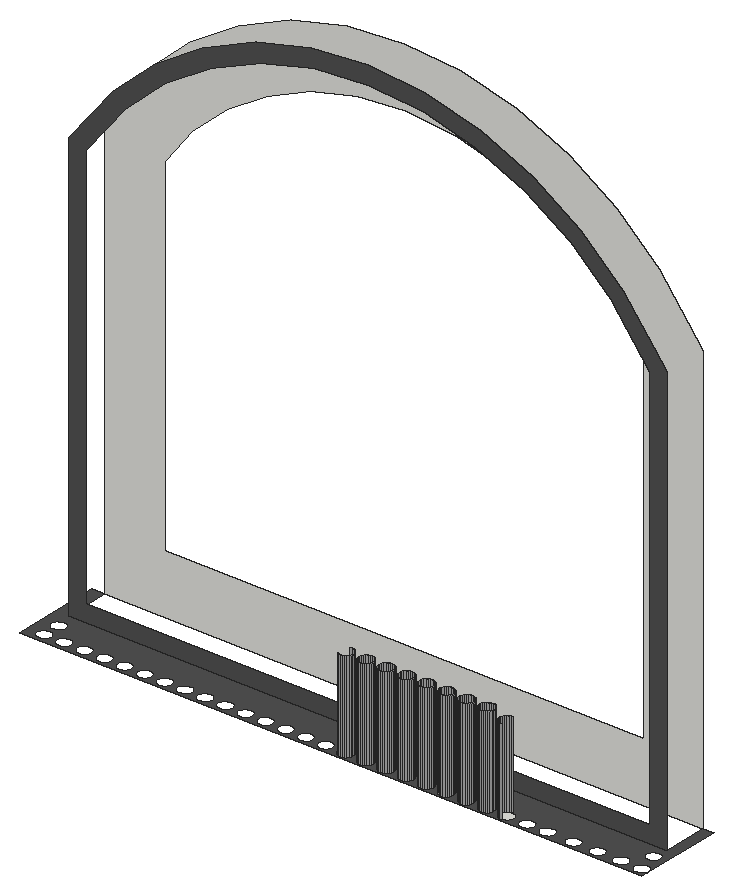
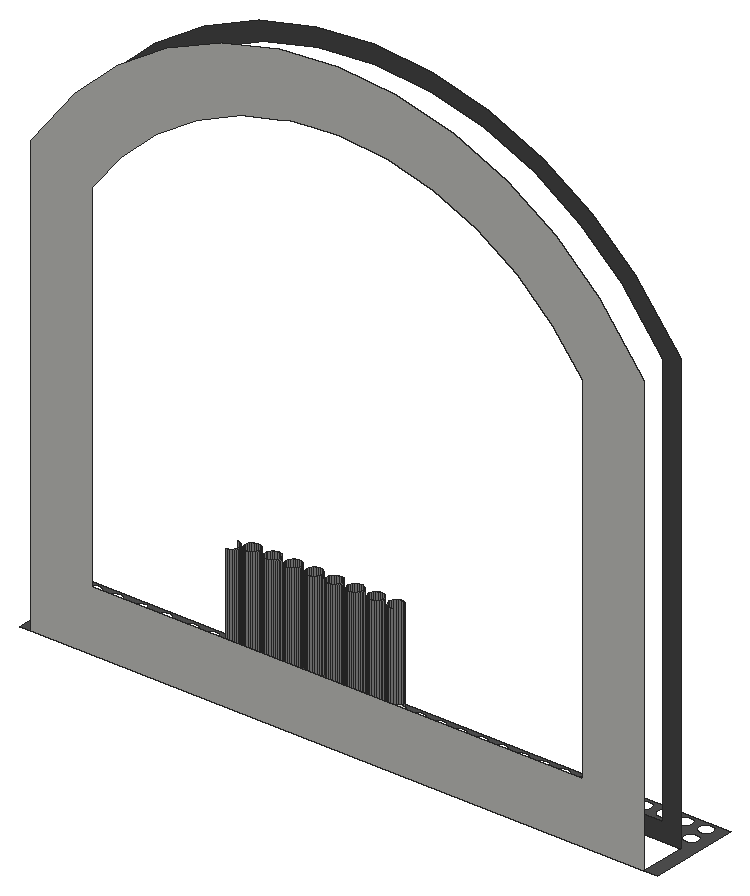
# SketchUp Ruby script. Lengths in inches.
U = 1.inch
M = Sketchup.active_model
def pt(a) = Geom::Point3d.new(a.map { |v| v * U })
def face(e, loops, mat)
  f = e.add_face(loops[0].map { |a| pt(a) })
  loops[1..].each { |l| e.add_face(l.map { |a| pt(a) }).erase! }
  f.material = f.back_material = mat if mat
  f
end
# faces: each face lists its corners as indices into pts; further lists are holes
def faces(e, pts, list, mat = nil) = list.each { |f| face(e, (f[0].is_a?(Array) ? f : [f]).map { |l| l.map { |i| pts[i] } }, mat) }
# xy, xz, yz: faces in a plane at the given z, y or x. An outline is a flat list of corners, or four numbers for a rectangle; further outlines are holes
def ring(l) = l.size == 4 ? [[l[0], l[1]], [l[2], l[1]], [l[2], l[3]], [l[0], l[3]]] : l.each_slice(2).to_a
def flat(e, list, mat, &to3) = list.each { |f| face(e, (f[0].is_a?(Array) ? f : [f]).map { |l| ring(l).map { |u, v| to3.(u, v) } }, mat) }
def xy(e, z, list, mat = nil) = flat(e, list, mat) { |x, y| [x, y, z] }
def xz(e, y, list, mat = nil) = flat(e, list, mat) { |x, z| [x, y, z] }
def yz(e, x, list, mat = nil) = flat(e, list, mat) { |y, z| [x, y, z] }
def lines(e, pts, list) = list.each { |a, b| e.add_line(pt(pts[a]), pt(pts[b])) }
# prism: a flat outline (further loops are holes) pulled along v
def prism(e, loops, v, mat = nil)
  f = face(e, loops, mat); d = Geom::Vector3d.new(v.map { |x| x * U })
  f.pushpull(f.normal.samedirection?(d) ? d.length : -d.length)
end
def box(e, o, s, mat = nil) = prism(e, [[o, [o[0] + s[0], o[1], o[2]], [o[0] + s[0], o[1] + s[1], o[2]], [o[0], o[1] + s[1], o[2]]]], [0, 0, s[2]], mat)
def at(x, y, z, deg = 0) = Geom::Transformation.translation(pt([x, y, z])) * Geom::Transformation.rotation(ORIGIN, Z_AXIS, deg.degrees)
def axes(o, x, y, z) = Geom::Transformation.new([*x, 0, *y, 0, *z, 0, *pt(o).to_a, 1])
def part(name) = M.definitions.add(name)
# library, detail: a bought-in or finely detailed component or shape, given as its bounding box
def library(name, o, s) = part(name).tap { |d| box(d.entities, o, s) }
def detail(e, o, s) = box(e.add_group.entities, o, s)
def put(e, d, t, mat = nil) = e.add_instance(d, t).tap { |i| i.material = mat if mat }
def group(e, t, mat = nil) = e.add_group.tap { |g| g.transformation = t; g.material = mat if mat }.entities
root = M.entities
M.materials.add("[0132_LightGray]").color = [169, 169, 169]
M.materials.add("[0135_DarkGray]").color = [81, 81, 81]
xy(root,180.28,[[302.06,32.09,301.6875,32.13,301.34,32.28,301.04,32.51,300.8125,32.8,300.67,33.15,300.62,33.52,300.67,33.89,300.8125,34.24,301.04,34.54,301.34,34.77,301.6875,34.91,302.06,34.96,302.43,34.91,302.78,34.77,303.08,34.54,303.3,34.24,303.45,33.89,303.5,33.52,303.45,33.15,303.3,32.8,303.08,32.51,302.78,32.28,302.43,32.13],[306.12,32.09,305.75,32.13,305.4,32.28,305.1,32.51,304.875,32.8,304.73,33.15,304.68,33.52,304.73,33.89,304.875,34.24,305.1,34.54,305.4,34.77,305.75,34.91,306.12,34.96,306.49,34.91,306.84,34.77,307.14,34.54,307.37,34.24,307.51,33.89,307.56,33.52,307.51,33.15,307.37,32.8,307.14,32.51,306.84,32.28,306.49,32.13],[310.18,32.09,309.8125,32.13,309.47,32.28,309.17,32.51,308.9375,32.8,308.8,33.15,308.75,33.52,308.8,33.89,308.9375,34.24,309.17,34.54,309.47,34.77,309.8125,34.91,310.18,34.96,310.56,34.91,310.9,34.77,311.2,34.54,311.43,34.24,311.57,33.89,311.62,33.52,311.57,33.15,311.43,32.8,311.2,32.51,310.9,32.28,310.56,32.13],[314.25,32.09,313.875,32.13,313.53,32.28,313.23,32.51,313,32.8,312.86,33.15,312.81,33.52,312.86,33.89,313,34.24,313.23,34.54,313.53,34.77,313.875,34.91,314.25,34.96,314.62,34.91,314.97,34.77,315.26,34.54,315.49,34.24,315.63,33.89,315.68,33.52,315.63,33.15,315.49,32.8,315.26,32.51,314.97,32.28,314.62,32.13],[318.31,32.09,317.9375,32.13,317.59,32.28,317.29,32.51,317.0625,32.8,316.92,33.15,316.87,33.52,316.92,33.89,317.0625,34.24,317.29,34.54,317.59,34.77,317.9375,34.91,318.31,34.96,318.68,34.91,319.03,34.77,319.33,34.54,319.55,34.24,319.7,33.89,319.75,33.52,319.7,33.15,319.55,32.8,319.33,32.51,319.03,32.28,318.68,32.13],
  [322.37,32.09,322,32.13,321.65,32.28,321.35,32.51,321.125,32.8,320.98,33.15,320.93,33.52,320.98,33.89,321.125,34.24,321.35,34.54,321.65,34.77,322,34.91,322.37,34.96,322.74,34.91,323.09,34.77,323.39,34.54,323.62,34.24,323.76,33.89,323.81,33.52,323.76,33.15,323.62,32.8,323.39,32.51,323.09,32.28,322.74,32.13],[326.43,32.09,326.0625,32.13,325.72,32.28,325.42,32.51,325.1875,32.8,325.05,33.15,325,33.52,325.05,33.89,325.1875,34.24,325.42,34.54,325.72,34.77,326.0625,34.91,326.43,34.96,326.81,34.91,327.15,34.77,327.45,34.54,327.68,34.24,327.82,33.89,327.87,33.52,327.82,33.15,327.68,32.8,327.45,32.51,327.15,32.28,326.81,32.13],[330.5,32.09,330.125,32.13,329.78,32.28,329.48,32.51,329.25,32.8,329.11,33.15,329.06,33.52,329.11,33.89,329.25,34.24,329.48,34.54,329.78,34.77,330.125,34.91,330.5,34.96,330.87,34.91,331.22,34.77,331.51,34.54,331.74,34.24,331.88,33.89,331.93,33.52,331.88,33.15,331.74,32.8,331.51,32.51,331.22,32.28,330.87,32.13],[334.56,32.09,334.1875,32.13,333.84,32.28,333.54,32.51,333.3125,32.8,333.17,33.15,333.12,33.52,333.17,33.89,333.3125,34.24,333.54,34.54,333.84,34.77,334.1875,34.91,334.56,34.96,334.93,34.91,335.28,34.77,335.58,34.54,335.8,34.24,335.95,33.89,336,33.52,335.95,33.15,335.8,32.8,335.58,32.51,335.28,32.28,334.93,32.13]])
xy(root,180.28,[[[237.76,31.6875,363.26,31.6875,363.26,49.6875,361.14,49.6875,361.14,40.6875,240.45,40.6875,240.45,49.6875,237.76,49.6875],[241.12,35.71,240.75,35.76,240.4,35.9,240.1,36.13,239.875,36.43,239.73,36.78,239.68,37.15,239.73,37.52,239.875,37.87,240.1,38.16,240.4,38.39,240.75,38.54,241.12,38.59,241.49,38.54,241.84,38.39,242.14,38.16,242.37,37.87,242.51,37.52,242.56,37.15,242.51,36.78,242.37,36.43,242.14,36.13,241.84,35.9,241.49,35.76],[241.12,32.09,240.75,32.13,240.4,32.28,240.1,32.51,239.875,32.8,239.73,33.15,239.68,33.52,239.73,33.89,239.875,34.24,240.1,34.54,240.4,34.77,240.75,34.91,241.12,34.96,241.49,34.91,241.84,34.77,242.14,34.54,242.37,34.24,242.51,33.89,242.56,33.52,242.51,33.15,242.37,32.8,242.14,32.51,241.84,32.28,241.49,32.13],[245.18,32.09,244.8125,32.13,244.47,32.28,244.17,32.51,243.9375,32.8,243.8,33.15,243.75,33.52,243.8,33.89,243.9375,34.24,244.17,34.54,244.47,34.77,244.8125,34.91,245.18,34.96,245.56,34.91,245.9,34.77,246.2,34.54,246.43,34.24,246.57,33.89,246.62,33.52,246.57,33.15,246.43,32.8,246.2,32.51,245.9,32.28,245.56,32.13],[249.25,32.09,248.875,32.13,248.53,32.28,248.23,32.51,248,32.8,247.86,33.15,247.81,33.52,247.86,33.89,248,34.24,248.23,34.54,248.53,34.77,248.875,34.91,249.25,34.96,249.62,34.91,249.97,34.77,250.26,34.54,250.49,34.24,250.63,33.89,250.68,33.52,250.63,33.15,250.49,32.8,250.26,32.51,249.97,32.28,249.62,32.13],[253.31,32.09,252.9375,32.13,252.59,32.28,252.29,32.51,252.0625,32.8,251.92,33.15,251.87,33.52,251.92,33.89,252.0625,34.24,252.29,34.54,252.59,34.77,252.9375,34.91,253.31,34.96,253.68,34.91,254.03,34.77,254.33,34.54,254.55,34.24,254.7,33.89,254.75,33.52,254.7,33.15,254.55,32.8,254.33,32.51,254.03,32.28,253.68,32.13],[257.37,32.09,257,32.13,256.65,32.28,256.35,32.51,256.125,32.8,255.98,33.15,255.93,33.52,255.98,33.89,256.125,34.24,256.35,34.54,256.65,34.77,257,34.91,257.37,34.96,257.74,34.91,258.09,34.77,258.39,34.54,258.62,34.24,258.76,33.89,258.81,33.52,258.76,33.15,258.62,32.8,258.39,32.51,258.09,32.28,257.74,32.13],[261.43,32.09,261.0625,32.13,260.72,32.28,260.42,32.51,260.1875,32.8,260.05,33.15,260,33.52,260.05,33.89,260.1875,34.24,260.42,34.54,260.72,34.77,261.0625,34.91,261.43,34.96,261.81,34.91,262.15,34.77,262.45,34.54,262.68,34.24,262.82,33.89,262.87,33.52,262.82,33.15,262.68,32.8,262.45,32.51,262.15,32.28,261.81,32.13],[265.5,32.09,265.125,32.13,264.78,32.28,264.48,32.51,264.25,32.8,264.11,33.15,264.06,33.52,264.11,33.89,264.25,34.24,264.48,34.54,264.78,34.77,265.125,34.91,265.5,34.96,265.87,34.91,266.22,34.77,266.51,34.54,266.74,34.24,266.88,33.89,266.93,33.52,266.88,33.15,266.74,32.8,266.51,32.51,266.22,32.28,265.87,32.13],[269.56,32.09,269.1875,32.13,268.84,32.28,268.54,32.51,268.3125,32.8,268.17,33.15,268.12,33.52,268.17,33.89,268.3125,34.24,268.54,34.54,268.84,34.77,269.1875,34.91,269.56,34.96,269.93,34.91,270.28,34.77,270.58,34.54,270.8,34.24,270.95,33.89,271,33.52,270.95,33.15,270.8,32.8,270.58,32.51,270.28,32.28,269.93,32.13],[273.62,32.09,273.25,32.13,272.9,32.28,272.6,32.51,272.375,32.8,272.23,33.15,272.18,33.52,272.23,33.89,272.375,34.24,272.6,34.54,272.9,34.77,273.25,34.91,273.62,34.96,273.99,34.91,274.34,34.77,274.64,34.54,274.87,34.24,275.01,33.89,275.06,33.52,275.01,33.15,274.87,32.8,274.64,32.51,274.34,32.28,273.99,32.13],[277.68,32.09,277.3125,32.13,276.97,32.28,276.67,32.51,276.4375,32.8,276.3,33.15,276.25,33.52,276.3,33.89,276.4375,34.24,276.67,34.54,276.97,34.77,277.3125,34.91,277.68,34.96,278.06,34.91,278.4,34.77,278.7,34.54,278.93,34.24,279.07,33.89,279.12,33.52,279.07,33.15,278.93,32.8,278.7,32.51,278.4,32.28,278.06,32.13],[281.75,32.09,281.375,32.13,281.03,32.28,280.73,32.51,280.5,32.8,280.36,33.15,280.31,33.52,280.36,33.89,280.5,34.24,280.73,34.54,281.03,34.77,281.375,34.91,281.75,34.96,282.12,34.91,282.47,34.77,282.76,34.54,282.99,34.24,283.13,33.89,283.18,33.52,283.13,33.15,282.99,32.8,282.76,32.51,282.47,32.28,282.12,32.13],[285.81,32.09,285.4375,32.13,285.09,32.28,284.79,32.51,284.5625,32.8,284.42,33.15,284.37,33.52,284.42,33.89,284.5625,34.24,284.79,34.54,285.09,34.77,285.4375,34.91,285.81,34.96,286.18,34.91,286.53,34.77,286.83,34.54,287.05,34.24,287.2,33.89,287.25,33.52,287.2,33.15,287.05,32.8,286.83,32.51,286.53,32.28,286.18,32.13],[289.87,32.09,289.5,32.13,289.15,32.28,288.85,32.51,288.625,32.8,288.48,33.15,288.43,33.52,288.48,33.89,288.625,34.24,288.85,34.54,289.15,34.77,289.5,34.91,289.87,34.96,290.24,34.91,290.59,34.77,290.89,34.54,291.12,34.24,291.26,33.89,291.31,33.52,291.26,33.15,291.12,32.8,290.89,32.51,290.59,32.28,290.24,32.13],[293.93,32.09,293.5625,32.13,293.22,32.28,292.92,32.51,292.6875,32.8,292.55,33.15,292.5,33.52,292.55,33.89,292.6875,34.24,292.92,34.54,293.22,34.77,293.5625,34.91,293.93,34.96,294.31,34.91,294.65,34.77,294.95,34.54,295.18,34.24,295.32,33.89,295.37,33.52,295.32,33.15,295.18,32.8,294.95,32.51,294.65,32.28,294.31,32.13],[298,32.09,297.625,32.13,297.28,32.28,296.98,32.51,296.75,32.8,296.61,33.15,296.56,33.52,296.61,33.89,296.75,34.24,296.98,34.54,297.28,34.77,297.625,34.91,298,34.96,298.37,34.91,298.72,34.77,299.01,34.54,299.24,34.24,299.38,33.89,299.43,33.52,299.38,33.15,299.24,32.8,299.01,32.51,298.72,32.28,298.37,32.13],[302.06,32.09,301.6875,32.13,301.34,32.28,301.04,32.51,300.8125,32.8,300.67,33.15,300.62,33.52,300.67,33.89,300.8125,34.24,301.04,34.54,301.34,34.77,301.6875,34.91,302.06,34.96,302.43,34.91,302.78,34.77,303.08,34.54,303.3,34.24,303.45,33.89,303.5,33.52,303.45,33.15,303.3,32.8,303.08,32.51,302.78,32.28,302.43,32.13],[306.12,32.09,305.75,32.13,305.4,32.28,305.1,32.51,304.875,32.8,304.73,33.15,304.68,33.52,304.73,33.89,304.875,34.24,305.1,34.54,305.4,34.77,305.75,34.91,306.12,34.96,306.49,34.91,306.84,34.77,307.14,34.54,307.37,34.24,307.51,33.89,307.56,33.52,307.51,33.15,307.37,32.8,307.14,32.51,306.84,32.28,306.49,32.13],[310.18,32.09,309.8125,32.13,309.47,32.28,309.17,32.51,308.9375,32.8,308.8,33.15,308.75,33.52,308.8,33.89,308.9375,34.24,309.17,34.54,309.47,34.77,309.8125,34.91,310.18,34.96,310.56,34.91,310.9,34.77,311.2,34.54,311.43,34.24,311.57,33.89,311.62,33.52,311.57,33.15,311.43,32.8,311.2,32.51,310.9,32.28,310.56,32.13],[314.25,32.09,313.875,32.13,313.53,32.28,313.23,32.51,313,32.8,312.86,33.15,312.81,33.52,312.86,33.89,313,34.24,313.23,34.54,313.53,34.77,313.875,34.91,314.25,34.96,314.62,34.91,314.97,34.77,315.26,34.54,315.49,34.24,315.63,33.89,315.68,33.52,315.63,33.15,315.49,32.8,315.26,32.51,314.97,32.28,314.62,32.13],[318.31,32.09,317.9375,32.13,317.59,32.28,317.29,32.51,317.0625,32.8,316.92,33.15,316.87,33.52,316.92,33.89,317.0625,34.24,317.29,34.54,317.59,34.77,317.9375,34.91,318.31,34.96,318.68,34.91,319.03,34.77,319.33,34.54,319.55,34.24,319.7,33.89,319.75,33.52,319.7,33.15,319.55,32.8,319.33,32.51,319.03,32.28,318.68,32.13],[322.37,32.09,322,32.13,321.65,32.28,321.35,32.51,321.125,32.8,320.98,33.15,320.93,33.52,320.98,33.89,321.125,34.24,321.35,34.54,321.65,34.77,322,34.91,322.37,34.96,322.74,34.91,323.09,34.77,323.39,34.54,323.62,34.24,323.76,33.89,323.81,33.52,323.76,33.15,323.62,32.8,323.39,32.51,323.09,32.28,322.74,32.13],[326.43,32.09,326.0625,32.13,325.72,32.28,325.42,32.51,325.1875,32.8,325.05,33.15,325,33.52,325.05,33.89,325.1875,34.24,325.42,34.54,325.72,34.77,326.0625,34.91,326.43,34.96,326.81,34.91,327.15,34.77,327.45,34.54,327.68,34.24,327.82,33.89,327.87,33.52,327.82,33.15,327.68,32.8,327.45,32.51,327.15,32.28,326.81,32.13],[330.5,32.09,330.125,32.13,329.78,32.28,329.48,32.51,329.25,32.8,329.11,33.15,329.06,33.52,329.11,33.89,329.25,34.24,329.48,34.54,329.78,34.77,330.125,34.91,330.5,34.96,330.87,34.91,331.22,34.77,331.51,34.54,331.74,34.24,331.88,33.89,331.93,33.52,331.88,33.15,331.74,32.8,331.51,32.51,331.22,32.28,330.87,32.13],[334.56,32.09,334.1875,32.13,333.84,32.28,333.54,32.51,333.3125,32.8,333.17,33.15,333.12,33.52,333.17,33.89,333.3125,34.24,333.54,34.54,333.84,34.77,334.1875,34.91,334.56,34.96,334.93,34.91,335.28,34.77,335.58,34.54,335.8,34.24,335.95,33.89,336,33.52,335.95,33.15,335.8,32.8,335.58,32.51,335.28,32.28,334.93,32.13],[338.62,32.09,338.25,32.13,337.9,32.28,337.6,32.51,337.375,32.8,337.23,33.15,337.18,33.52,337.23,33.89,337.375,34.24,337.6,34.54,337.9,34.77,338.25,34.91,338.62,34.96,338.99,34.91,339.34,34.77,339.64,34.54,339.87,34.24,340.01,33.89,340.06,33.52,340.01,33.15,339.87,32.8,339.64,32.51,339.34,32.28,338.99,32.13],[342.68,32.09,342.3125,32.13,341.97,32.28,341.67,32.51,341.4375,32.8,341.3,33.15,341.25,33.52,341.3,33.89,341.4375,34.24,341.67,34.54,341.97,34.77,342.3125,34.91,342.68,34.96,343.06,34.91,343.4,34.77,343.7,34.54,343.93,34.24,344.07,33.89,344.12,33.52,344.07,33.15,343.93,32.8,343.7,32.51,343.4,32.28,343.06,32.13],[347.93,32.09,347.5625,32.13,347.22,32.28,346.92,32.51,346.6875,32.8,346.55,33.15,346.5,33.52,346.55,33.89,346.6875,34.24,346.92,34.54,347.22,34.77,347.5625,34.91,347.93,34.96,348.31,34.91,348.65,34.77,348.95,34.54,349.18,34.24,349.32,33.89,349.37,33.52,349.32,33.15,349.18,32.8,348.95,32.51,348.65,32.28,348.31,32.13],[352.81,32.09,352.4375,32.13,352.09,32.28,351.79,32.51,351.5625,32.8,351.42,33.15,351.37,33.52,351.42,33.89,351.5625,34.24,351.79,34.54,352.09,34.77,352.4375,34.91,352.81,34.96,353.18,34.91,353.53,34.77,353.83,34.54,354.05,34.24,354.2,33.89,354.25,33.52,354.2,33.15,354.05,32.8,353.83,32.51,353.53,32.28,353.18,32.13],[357.56,32.09,357.1875,32.13,356.84,32.28,356.54,32.51,356.3125,32.8,356.17,33.15,356.12,33.52,356.17,33.89,356.3125,34.24,356.54,34.54,356.84,34.77,357.1875,34.91,357.56,34.96,357.93,34.91,358.28,34.77,358.58,34.54,358.8,34.24,358.95,33.89,359,33.52,358.95,33.15,358.8,32.8,358.58,32.51,358.28,32.28,357.93,32.13],[361.68,32.09,361.3125,32.13,360.97,32.28,360.67,32.51,360.4375,32.8,360.3,33.15,360.25,33.52,360.3,33.89,360.4375,34.24,360.67,34.54,360.97,34.77,361.3125,34.91,361.68,34.96,362.06,34.91,362.4,34.77,362.7,34.54,362.93,34.24,363.07,33.89,363.12,33.52,363.07,33.15,362.93,32.8,362.7,32.51,362.4,32.28,362.06,32.13],[360.7,36.35,360.32,36.4,359.98,36.54,359.68,36.77,359.45,37.07,359.31,37.41,359.26,37.78,359.31,38.16,359.45,38.5,359.68,38.8,359.98,39.03,360.32,39.17,360.7,39.22,361.07,39.17,361.41,39.03,361.71,38.8,361.94,38.5,362.08,38.16,362.13,37.78,362.08,37.41,361.94,37.07,361.71,36.77,361.41,36.54,361.07,36.4]]],"[0135_DarkGray]")
xz(root,40.6875,[[[240.45,180.28,361.14,180.28,361.14,266.7,352.21,278.3,343.74,286.17,334.09,292.53,323.51,297.2,312.3125,300.05,300.79,301.01,289.27,300.05,278.07,297.2,267.5,292.53,257.84,286.17,249.375,278.3,240.45,266.7],[243.9,183.73,243.9,265.52,251.94,275.97,259.98,283.44,269.16,289.48,279.2,293.92,289.85,296.64,300.79,297.55,311.74,296.64,322.38,293.92,332.43,289.48,341.6,283.44,349.65,275.97,357.68,265.52,357.68,183.73]]],"[0135_DarkGray]")
xz(root,49.6875,[[[240.45,180.28,240.45,266.7,249.375,278.3,257.84,286.17,267.5,292.53,278.07,297.2,289.27,300.05,300.79,301.01,312.3125,300.05,323.51,297.2,334.09,292.53,343.74,286.17,352.21,278.3,361.14,266.7,361.14,180.28],[252.45,192.28,349.14,192.28,349.14,262.62,343.31,270.19,336.3,276.7,328.32,281.95,319.58,285.82,311.64,287.84,310.32,288.18,305.64,288.57,300.79,288.97,291.27,288.18,282,285.82,273.26,281.95,265.28,276.7,258.28,270.19,252.45,262.62]]])
p = [[301.34,32.28,180.28],[301.6875,32.13,180.28],[301.6875,32.13,198.6],[301.34,32.28,198.6],[302.06,32.09,180.28],[302.06,32.09,198.6],
  [302.43,32.13,180.28],[302.43,32.13,198.6],[302.78,32.28,180.28],[302.78,32.28,198.6],[305.4,32.28,180.28],[305.75,32.13,180.28],
  [305.75,32.13,198.6],[305.4,32.28,198.6],[306.12,32.09,180.28],[306.12,32.09,198.6],[306.49,32.13,180.28],[306.49,32.13,198.6],
  [306.84,32.28,180.28],[306.84,32.28,198.6],[309.47,32.28,180.28],[309.8125,32.13,180.28],[309.8125,32.13,198.6],[309.47,32.28,198.6],
  [310.18,32.09,180.28],[310.18,32.09,198.6],[310.56,32.13,180.28],[310.56,32.13,198.6],[310.9,32.28,180.28],[310.9,32.28,198.6],
  [313.53,32.28,180.28],[313.875,32.13,180.28],[313.875,32.13,198.6],[313.53,32.28,198.6],[314.25,32.09,180.28],[314.25,32.09,198.6],
  [314.62,32.13,180.28],[314.62,32.13,198.6],[314.97,32.28,180.28],[314.97,32.28,198.6],[317.59,32.28,180.28],[317.9375,32.13,180.28],
  [317.9375,32.13,198.6],[317.59,32.28,198.6],[318.31,32.09,180.28],[318.31,32.09,198.6],[318.68,32.13,180.28],[318.68,32.13,198.6],
  [319.03,32.28,180.28],[319.03,32.28,198.6],[321.65,32.28,180.28],[322,32.13,180.28],[322,32.13,198.6],[321.65,32.28,198.6],
  [322.37,32.09,180.28],[322.37,32.09,198.6],[322.74,32.13,180.28],[322.74,32.13,198.6],[323.09,32.28,180.28],[323.09,32.28,198.6],
  [325.72,32.28,180.28],[326.0625,32.13,180.28],[326.0625,32.13,198.6],[325.72,32.28,198.6],[326.43,32.09,180.28],[326.43,32.09,198.6],
  [326.81,32.13,180.28],[326.81,32.13,198.6],[327.15,32.28,180.28],[327.15,32.28,198.6],[329.78,32.28,180.28],[330.125,32.13,180.28],
  [330.125,32.13,198.6],[329.78,32.28,198.6],[330.5,32.09,180.28],[330.5,32.09,198.6],[330.87,32.13,180.28],[330.87,32.13,198.6],
  [331.22,32.28,180.28],[331.22,32.28,198.6],[333.84,32.28,180.28],[334.1875,32.13,180.28],[334.1875,32.13,197.66],[333.84,32.28,197.66],
  [334.56,32.09,180.28],[334.56,32.09,197.66],[303.08,32.51,180.28],[303.08,32.51,198.6],[305.1,32.51,180.28],[305.1,32.51,198.6],
  [307.14,32.51,180.28],[307.14,32.51,198.6],[309.17,32.51,180.28],[309.17,32.51,198.6],[311.2,32.51,180.28],[311.2,32.51,198.6],
  [313.23,32.51,180.28],[313.23,32.51,198.6],[315.26,32.51,180.28],[315.26,32.51,198.6],[317.29,32.51,180.28],[317.29,32.51,198.6],
  [319.33,32.51,180.28],[319.33,32.51,198.6],[321.35,32.51,180.28],[321.35,32.51,198.6],[323.39,32.51,180.28],[323.39,32.51,198.6],
  [325.42,32.51,180.28],[325.42,32.51,198.6],[327.45,32.51,180.28],[327.45,32.51,198.6],[329.48,32.51,180.28],[329.48,32.51,198.6],
  [331.51,32.51,180.28],[331.51,32.51,198.6],[333.54,32.51,180.28],[333.54,32.51,197.66],[303.3,32.8,180.28],[303.3,32.8,198.6],
  [304.875,32.8,180.28],[304.875,32.8,198.6],[307.37,32.8,180.28],[307.37,32.8,198.6],[308.9375,32.8,180.28],[308.9375,32.8,198.6],
  [311.43,32.8,180.28],[311.43,32.8,198.6],[313,32.8,180.28],[313,32.8,198.6],[315.49,32.8,180.28],[315.49,32.8,198.6],
  [317.0625,32.8,180.28],[317.0625,32.8,198.6],[319.55,32.8,180.28],[319.55,32.8,198.6],[321.125,32.8,180.28],[321.125,32.8,198.6],
  [323.62,32.8,180.28],[323.62,32.8,198.6],[325.1875,32.8,180.28],[325.1875,32.8,198.6],[327.68,32.8,180.28],[327.68,32.8,198.6],
  [329.25,32.8,180.28],[329.25,32.8,198.6],[331.74,32.8,180.28],[331.74,32.8,198.6],[333.3125,32.8,180.28],[333.3125,32.8,197.66],
  [303.45,33.15,180.28],[303.45,33.15,198.6],[304.73,33.15,180.28],[304.73,33.15,198.6],[307.51,33.15,180.28],[307.51,33.15,198.6],
  [308.8,33.15,180.28],[308.8,33.15,198.6],[311.57,33.15,180.28],[311.57,33.15,198.6],[312.86,33.15,180.28],[312.86,33.15,198.6],
  [315.63,33.15,180.28],[315.63,33.15,198.6],[316.92,33.15,180.28],[316.92,33.15,198.6],[319.7,33.15,180.28],[319.7,33.15,198.6],
  [320.98,33.15,180.28],[320.98,33.15,198.6],[323.76,33.15,180.28],[323.76,33.15,198.6],[325.05,33.15,180.28],[325.05,33.15,198.6],
  [327.82,33.15,180.28],[327.82,33.15,198.6],[329.11,33.15,180.28],[329.11,33.15,198.6],[331.88,33.15,180.28],[331.88,33.15,198.6],
  [333.17,33.15,180.28],[333.17,33.15,197.66],[303.5,33.52,180.28],[303.5,33.52,198.6],[304.68,33.52,180.28],[304.68,33.52,198.6],
  [307.56,33.52,180.28],[307.56,33.52,198.6],[308.75,33.52,180.28],[308.75,33.52,198.6],[311.62,33.52,180.28],[311.62,33.52,198.6],
  [312.81,33.52,180.28],[312.81,33.52,198.6],[315.68,33.52,180.28],[315.68,33.52,198.6],[316.87,33.52,180.28],[316.87,33.52,198.6],
  [319.75,33.52,180.28],[319.75,33.52,198.6],[320.93,33.52,180.28],[320.93,33.52,198.6],[323.81,33.52,180.28],[323.81,33.52,198.6],
  [325,33.52,180.28],[325,33.52,198.6],[327.87,33.52,180.28],[327.87,33.52,198.6],[329.06,33.52,180.28],[329.06,33.52,198.6],
  [331.93,33.52,180.28],[331.93,33.52,198.6],[333.12,33.52,180.28],[333.12,33.52,197.66],[303.45,33.89,180.28],[303.45,33.89,198.6],
  [304.73,33.89,180.28],[304.73,33.89,198.6],[307.51,33.89,180.28],[307.51,33.89,198.6],[308.8,33.89,180.28],[308.8,33.89,198.6],
  [311.57,33.89,180.28],[311.57,33.89,198.6],[312.86,33.89,180.28],[312.86,33.89,198.6],[315.63,33.89,180.28],[315.63,33.89,198.6],
  [316.92,33.89,180.28],[316.92,33.89,198.6],[319.7,33.89,180.28],[319.7,33.89,198.6],[320.98,33.89,180.28],[320.98,33.89,198.6],
  [323.76,33.89,180.28],[323.76,33.89,198.6],[325.05,33.89,180.28],[325.05,33.89,198.6],[327.82,33.89,180.28],[327.82,33.89,198.6],
  [329.11,33.89,180.28],[329.11,33.89,198.6],[331.88,33.89,180.28],[331.88,33.89,198.6],[333.17,33.89,180.28],[333.17,33.89,197.66],
  [303.3,34.24,180.28],[303.3,34.24,198.6],[304.875,34.24,180.28],[304.875,34.24,198.6],[307.37,34.24,180.28],[307.37,34.24,198.6],
  [308.9375,34.24,180.28],[308.9375,34.24,198.6],[311.43,34.24,180.28],[311.43,34.24,198.6],[313,34.24,180.28],[313,34.24,198.6],
  [315.49,34.24,180.28],[315.49,34.24,198.6],[317.0625,34.24,180.28],[317.0625,34.24,198.6],[319.55,34.24,180.28],[319.55,34.24,198.6],
  [321.125,34.24,180.28],[321.125,34.24,198.6],[323.62,34.24,180.28],[323.62,34.24,198.6],[325.1875,34.24,180.28],[325.1875,34.24,198.6],
  [327.68,34.24,180.28],[327.68,34.24,198.6],[329.25,34.24,180.28],[329.25,34.24,198.6],[331.74,34.24,180.28],[331.74,34.24,198.6],
  [333.3125,34.24,180.28],[333.3125,34.24,197.66],[303.08,34.54,180.28],[303.08,34.54,198.6],[305.1,34.54,180.28],[305.1,34.54,198.6],
  [307.14,34.54,180.28],[307.14,34.54,198.6],[309.17,34.54,180.28],[309.17,34.54,198.6],[311.2,34.54,180.28],[311.2,34.54,198.6],
  [313.23,34.54,180.28],[313.23,34.54,198.6],[315.26,34.54,180.28],[315.26,34.54,198.6],[317.29,34.54,180.28],[317.29,34.54,198.6],
  [319.33,34.54,180.28],[319.33,34.54,198.6],[321.35,34.54,180.28],[321.35,34.54,198.6],[323.39,34.54,180.28],[323.39,34.54,198.6],
  [325.42,34.54,180.28],[325.42,34.54,198.6],[327.45,34.54,180.28],[327.45,34.54,198.6],[329.48,34.54,180.28],[329.48,34.54,198.6],
  [331.51,34.54,180.28],[331.51,34.54,198.6],[333.54,34.54,180.28],[333.54,34.54,197.66],[302.78,34.77,180.28],[302.78,34.77,198.6],
  [305.4,34.77,180.28],[305.4,34.77,198.6],[306.84,34.77,180.28],[306.84,34.77,198.6],[309.47,34.77,180.28],[309.47,34.77,198.6],
  [310.9,34.77,180.28],[310.9,34.77,198.6],[313.53,34.77,180.28],[313.53,34.77,198.6],[314.97,34.77,180.28],[314.97,34.77,198.6],
  [317.59,34.77,180.28],[317.59,34.77,198.6],[319.03,34.77,180.28],[319.03,34.77,198.6],[321.65,34.77,180.28],[321.65,34.77,198.6],
  [323.09,34.77,180.28],[323.09,34.77,198.6],[325.72,34.77,180.28],[325.72,34.77,198.6],[327.15,34.77,180.28],[327.15,34.77,198.6],
  [329.78,34.77,180.28],[329.78,34.77,198.6],[331.22,34.77,180.28],[331.22,34.77,198.6],[333.84,34.77,180.28],[333.84,34.77,197.66],
  [302.43,34.91,180.28],[302.43,34.91,198.6],[305.75,34.91,180.28],[305.75,34.91,198.6],[306.49,34.91,180.28],[306.49,34.91,198.6],
  [309.8125,34.91,180.28],[309.8125,34.91,198.6],[310.56,34.91,180.28],[310.56,34.91,198.6],[313.875,34.91,180.28],[313.875,34.91,198.6],
  [314.62,34.91,180.28],[314.62,34.91,198.6],[317.9375,34.91,180.28],[317.9375,34.91,198.6],[318.68,34.91,180.28],[318.68,34.91,198.6],
  [322,34.91,180.28],[322,34.91,198.6],[322.74,34.91,180.28],[322.74,34.91,198.6],[326.0625,34.91,180.28],[326.0625,34.91,198.6],
  [326.81,34.91,180.28],[326.81,34.91,198.6],[330.125,34.91,180.28],[330.125,34.91,198.6],[330.87,34.91,180.28],[330.87,34.91,198.6],
  [334.1875,34.91,180.28],[334.1875,34.91,197.66],[302.06,34.96,180.28],[301.6875,34.91,180.28],[301.6875,34.91,198.6],[302.06,34.96,198.6],
  [306.12,34.96,180.28],[306.12,34.96,198.6],[310.18,34.96,180.28],[310.18,34.96,198.6],[314.25,34.96,180.28],[314.25,34.96,198.6],
  [318.31,34.96,180.28],[318.31,34.96,198.6],[322.37,34.96,180.28],[322.37,34.96,198.6],[326.43,34.96,180.28],[326.43,34.96,198.6],
  [330.5,34.96,180.28],[330.5,34.96,198.6],[334.56,34.96,180.28],[334.56,34.96,197.66]]
faces(root,p,[[0,1,2,3],[1,4,5,2],[4,6,7,5],[6,8,9,7],[10,11,12,13],[11,14,15,12],[14,16,17,15],[16,18,19,17],
  [20,21,22,23],[21,24,25,22],[24,26,27,25],[26,28,29,27],[30,31,32,33],[31,34,35,32],[34,36,37,35],[36,38,39,37],
  [40,41,42,43],[41,44,45,42],[44,46,47,45],[46,48,49,47],[50,51,52,53],[51,54,55,52],[54,56,57,55],[56,58,59,57],
  [60,61,62,63],[61,64,65,62],[64,66,67,65],[66,68,69,67],[70,71,72,73],[71,74,75,72],[74,76,77,75],[76,78,79,77],
  [80,81,82,83],[81,84,85,82],[8,86,87,9],[88,10,13,89],[18,90,91,19],[92,20,23,93],[28,94,95,29],[96,30,33,97],
  [38,98,99,39],[100,40,43,101],[48,102,103,49],[104,50,53,105],[58,106,107,59],[108,60,63,109],[68,110,111,69],[112,70,73,113],
  [78,114,115,79],[116,80,83,117],[86,118,119,87],[120,88,89,121],[90,122,123,91],[124,92,93,125],[94,126,127,95],[128,96,97,129],
  [98,130,131,99],[132,100,101,133],[102,134,135,103],[136,104,105,137],[106,138,139,107],[140,108,109,141],[110,142,143,111],[144,112,113,145],
  [114,146,147,115],[148,116,117,149],[118,150,151,119],[152,120,121,153],[122,154,155,123],[156,124,125,157],[126,158,159,127],[160,128,129,161],
  [130,162,163,131],[164,132,133,165],[134,166,167,135],[168,136,137,169],[138,170,171,139],[172,140,141,173],[142,174,175,143],[176,144,145,177],
  [146,178,179,147],[180,148,149,181],[150,182,183,151],[184,152,153,185],[154,186,187,155],[188,156,157,189],[158,190,191,159],[192,160,161,193],
  [162,194,195,163],[196,164,165,197],[166,198,199,167],[200,168,169,201],[170,202,203,171],[204,172,173,205],[174,206,207,175],[208,176,177,209],
  [178,210,211,179],[212,180,181,213],[182,214,215,183],[216,184,185,217],[186,218,219,187],[220,188,189,221],[190,222,223,191],[224,192,193,225],
  [194,226,227,195],[228,196,197,229],[198,230,231,199],[232,200,201,233],[202,234,235,203],[236,204,205,237],[206,238,239,207],[240,208,209,241],
  [210,242,243,211],[244,212,213,245],[214,246,247,215],[248,216,217,249],[218,250,251,219],[252,220,221,253],[222,254,255,223],[256,224,225,257],
  [226,258,259,227],[260,228,229,261],[230,262,263,231],[264,232,233,265],[234,266,267,235],[268,236,237,269],[238,270,271,239],[272,240,241,273],
  [242,274,275,243],[276,244,245,277],[246,278,279,247],[280,248,249,281],[250,282,283,251],[284,252,253,285],[254,286,287,255],[288,256,257,289],
  [258,290,291,259],[292,260,261,293],[262,294,295,263],[296,264,265,297],[266,298,299,267],[300,268,269,301],[270,302,303,271],[304,272,273,305],
  [274,306,307,275],[308,276,277,309],[278,310,311,279],[312,280,281,313],[282,314,315,283],[316,284,285,317],[286,318,319,287],[320,288,289,321],
  [290,322,323,291],[324,292,293,325],[294,326,327,295],[328,296,297,329],[298,330,331,299],[332,300,301,333],[302,334,335,303],[336,304,305,337],
  [306,338,339,307],[340,308,309,341],[310,342,343,311],[344,312,313,345],[314,346,347,315],[348,316,317,349],[318,350,351,319],[352,320,321,353],
  [322,354,355,323],[356,324,325,357],[326,358,359,327],[360,328,329,361],[330,362,363,331],[364,332,333,365],[334,366,367,335],[368,336,337,369],
  [338,370,371,339],[372,340,341,373],[374,375,376,377],[342,374,377,343],[378,344,345,379],[346,378,379,347],[380,348,349,381],[350,380,381,351],
  [382,352,353,383],[354,382,383,355],[384,356,357,385],[358,384,385,359],[386,360,361,387],[362,386,387,363],[388,364,365,389],[366,388,389,367],
  [390,368,369,391],[370,390,391,371],[392,372,373,393]],"[0132_LightGray]")
